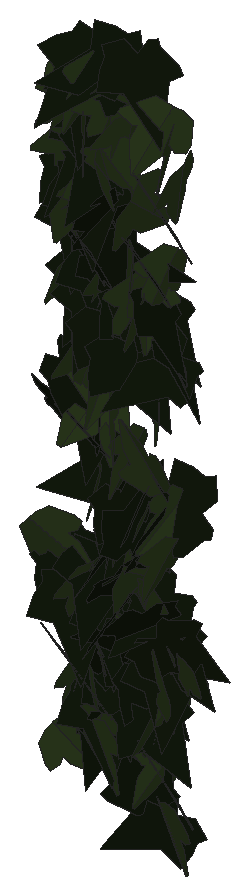
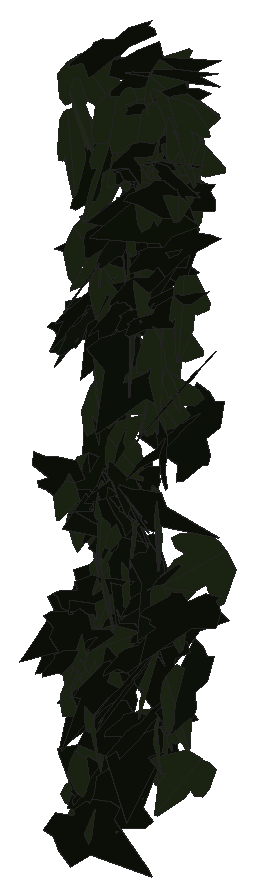
# SketchUp Ruby script. Lengths in inches.
U = 1.inch
M = Sketchup.active_model
def pt(a) = Geom::Point3d.new(a.map { |v| v * U })
def face(e, loops, mat)
  f = e.add_face(loops[0].map { |a| pt(a) })
  loops[1..].each { |l| e.add_face(l.map { |a| pt(a) }).erase! }
  f.material = f.back_material = mat if mat
  f
end
# faces: each face lists its corners as indices into pts; further lists are holes
def faces(e, pts, list, mat = nil) = list.each { |f| face(e, (f[0].is_a?(Array) ? f : [f]).map { |l| l.map { |i| pts[i] } }, mat) }
# xy, xz, yz: faces in a plane at the given z, y or x. An outline is a flat list of corners, or four numbers for a rectangle; further outlines are holes
def ring(l) = l.size == 4 ? [[l[0], l[1]], [l[2], l[1]], [l[2], l[3]], [l[0], l[3]]] : l.each_slice(2).to_a
def flat(e, list, mat, &to3) = list.each { |f| face(e, (f[0].is_a?(Array) ? f : [f]).map { |l| ring(l).map { |u, v| to3.(u, v) } }, mat) }
def xy(e, z, list, mat = nil) = flat(e, list, mat) { |x, y| [x, y, z] }
def xz(e, y, list, mat = nil) = flat(e, list, mat) { |x, z| [x, y, z] }
def yz(e, x, list, mat = nil) = flat(e, list, mat) { |y, z| [x, y, z] }
def lines(e, pts, list) = list.each { |a, b| e.add_line(pt(pts[a]), pt(pts[b])) }
# prism: a flat outline (further loops are holes) pulled along v
def prism(e, loops, v, mat = nil)
  f = face(e, loops, mat); d = Geom::Vector3d.new(v.map { |x| x * U })
  f.pushpull(f.normal.samedirection?(d) ? d.length : -d.length)
end
def box(e, o, s, mat = nil) = prism(e, [[o, [o[0] + s[0], o[1], o[2]], [o[0] + s[0], o[1] + s[1], o[2]], [o[0], o[1] + s[1], o[2]]]], [0, 0, s[2]], mat)
def at(x, y, z, deg = 0) = Geom::Transformation.translation(pt([x, y, z])) * Geom::Transformation.rotation(ORIGIN, Z_AXIS, deg.degrees)
def axes(o, x, y, z) = Geom::Transformation.new([*x, 0, *y, 0, *z, 0, *pt(o).to_a, 1])
def part(name) = M.definitions.add(name)
# library, detail: a bought-in or finely detailed component or shape, given as its bounding box
def library(name, o, s) = part(name).tap { |d| box(d.entities, o, s) }
def detail(e, o, s) = box(e.add_group.entities, o, s)
def put(e, d, t, mat = nil) = e.add_instance(d, t).tap { |i| i.material = mat if mat }
def group(e, t, mat = nil) = e.add_group.tap { |g| g.transformation = t; g.material = mat if mat }.entities
root = M.entities
M.materials.add("efeu1").color = [18, 25, 13]
M.materials.add("efeu2").color = [43, 57, 29]
c1 = part("ivyleaf_10")
p = [[0,0.5,-0.03],[-0.0625,2.02,-0.43],[-0.19,2.01,-0.46],[-0.54,1.05,-0.29],[-0.52,0.625,-0.18],[-0.83,0.76,-0.28],
  [-1.16,0.64,-0.33],[-1.15,0.33,-0.24],[-0.77,-0.39,0.02],[-0.3,-0.51,0.16],[0.04,-0.48,0.23],[-0.02,2.01,-0.4375],
  [-0.06,2.01,-0.43],[0.04,-0.49,0.23],[0.67,-0.49,0.14],[1.38,0.36,-0.2],[1.375,0.51,-0.24],[0.81,0.65,-0.19],
  [0.62,0.59,-0.15],[0.6,1.09,-0.28],[0.5,1.23,-0.31]]
faces(c1.entities,p,[[0,1,2,3,4,5,6,7,8,9,10],[11,12,0,13,14,15,16,17,18,19,20]],"efeu2")
c2 = part("ivyleaf_9")
p = [[1.54,2.16,1.25],[1.36,2.04,1.19],[-0.21,0.99,0.68],[-0.71,1.11,0.82],[-0.85,0.86,0.67],[-0.8,0.17,0.21],
  [-0.9,-0.01,0.1],[-0.67,-0.16,-0.02],[-0.08,-0.08,-0.05],[-0.03,-0.6,-0.4],[0.65,-0.88,-0.66],[0.83,-0.6,-0.49],
  [1.29,-0.42,-0.43],[1.8125,-0.07,-0.26],[1.21,0.44,0.15]]
faces(c2.entities,p,[[0,1,2,3,4,5,6,7,8,9,10,11,12,13,14]],"efeu1")
put(root,c1,axes([527.49,134.28,199.55],[0.10331,-0.77036,-0.31589],[0.02742,0.32128,-0.77456],[0.83216,0.08505,0.06474]))
put(root,c1,axes([527.53,134.26,204.45],[0.00296,-0.85137,0.05429],[0.01786,-0.05421,-0.85119],[0.85291,0.00408,0.01763]))
put(root,c1,axes([527.09,133.73,191.82],[-0.55023,-0.01152,-0.61627],[0.61539,0.03637,-0.55013],[0.0348,-0.82536,-0.01563]))
put(root,c2,axes([527.21,134.57,190.82],[0.02669,-0.53096,-0.58579],[0.07368,0.58524,-0.5271],[0.78717,-0.03678,0.0692]))
put(root,c1,axes([527.72,134.58,204.76],[-0.5819,-0.55056,0.2142],[-0.09039,-0.21415,-0.79598],[0.58381,-0.58192,0.09026]))
put(root,c1,axes([527.43,134.8,205.12],[0.84438,-0.03795,0.0025],[0.00327,0.01701,-0.84506],[0.03789,0.84422,0.01714]))
put(root,c1,axes([527.77,134.18,203.35],[-0.60526,-0.56127,0.00643],[-0.00507,-0.00399,-0.82544],[0.56128,-0.60528,-0.00052]))
put(root,c1,axes([527.49,133.99,185.72],[0.32694,0.47097,0.47558],[0.1738,0.4514,-0.5665],[-0.64636,0.3596,0.08824]))
put(root,c2,axes([527.64,134.87,201.06],[-0.28917,-0.75904,-0.0645],[0.0197,0.06152,-0.81225],[0.76152,-0.28981,-0.00348]))
put(root,c2,axes([527.11,134.03,195.4],[0.59961,-0.41124,0.45427],[0.37216,-0.26053,-0.72708],[0.48681,0.70571,-0.0037]))
put(root,c1,axes([527.89,134.27,187.93],[0.213,-0.80801,0.14369],[0.05539,-0.13396,-0.83539],[0.81881,0.21925,0.01913]))
put(root,c2,axes([527.89,135,199.15],[-0.33172,-0.70773,0.18093],[-0.02622,-0.18705,-0.77973],[0.73002,-0.32831,0.05421]))
put(root,c2,axes([527.34,134.16,188.06],[0.53366,-0.51151,0.41089],[0.28566,-0.29567,-0.73909],[0.59065,0.60515,-0.0138]))
put(root,c2,axes([527.65,133.8,196.87],[0.5477,-0.49041,-0.45193],[-0.19676,0.43995,-0.71585],[0.6372,0.55737,0.16741]))
put(root,c2,axes([527.68,134.5,202.52],[-0.11047,-0.63485,-0.51519],[0.22003,0.47761,-0.63572],[0.78743,-0.22252,0.10536]))
put(root,c1,axes([528.34,134.28,186.85],[-0.07324,0.12878,-0.83192],[-0.32133,0.76756,0.14711],[0.77809,0.32911,-0.01755]))
put(root,c1,axes([528.1875,134.55,193.38],[0.34283,-0.596,-0.44686],[-0.15045,0.42638,-0.6841],[0.72956,0.368,0.06891]))
put(root,c2,axes([527.83,134.27,190],[-0.22233,-0.79633,-0.23959],[0.10442,0.21931,-0.82582],[0.82501,-0.24236,0.03995]))
put(root,c2,axes([528.625,134.9,193.3125],[-0.61958,0.04282,0.46131],[-0.46161,0.00845,-0.62077],[-0.0394,-0.77241,0.01878]))
put(root,c2,axes([528.22,134.72,203.05],[-0.78111,-0.17497,-0.20759],[0.20422,0.03799,-0.80043],[0.1789,-0.80733,0.00732]))
put(root,c2,axes([528.2,134.53,205.75],[-0.69733,-0.48736,0.10601],[0.07458,-0.28207,-0.80617],[0.49315,-0.64649,0.27182]))
put(root,c1,axes([528.1875,134.14,190.65],[0.02802,-0.80758,0.08612],[-0.00555,-0.08636,-0.80803],[0.81214,0.02727,-0.00849]))
put(root,c2,axes([528.42,134.15,194.625],[0.04968,-0.09958,0.80488],[-0.177,0.78562,0.10812],[-0.79146,-0.18194,0.02634]))
put(root,c2,axes([527.92,134.94,203.9375],[-0.17494,-0.77201,-0.2741],[0.06505,0.2663,-0.79157],[0.81664,-0.18659,0.00434]))
put(root,c2,axes([527.87,134.95,195.23],[-0.03168,-0.79066,0.24981],[0.03349,-0.25101,-0.7902],[0.82851,-0.02008,0.0415]))
put(root,c1,axes([528.06,134.42,204.07],[-0.18171,0.64404,-0.48709],[0.08272,-0.4818,-0.6679],[-0.80325,-0.19531,0.04141]))
put(root,c2,axes([528.11,134.74,205],[-0.3204,-0.76889,-0.04698],[0.00681,0.04805,-0.83289],[0.77029,-0.32024,-0.01217]))
put(root,c1,axes([528.39,134.98,204.6],[-0.41538,-0.68563,0.16225],[-0.05821,-0.1543,-0.8011],[0.70216,-0.4184,0.02957]))
put(root,c2,axes([528.38,134.74,203],[-0.66306,-0.47663,0.15068],[-0.00707,-0.24134,-0.7945],[0.49983,-0.6357,0.18866]))
put(root,c1,axes([528.22,134.37,205.36],[0.01143,-0.59414,0.59444],[0.14879,-0.58367,-0.58624],[0.82718,0.1132,0.09724]))
put(root,c1,axes([528.4,134.3,202.2],[-0.13464,-0.76169,0.27538],[-0.05587,-0.26975,-0.77346],[0.80801,-0.14557,-0.0076]))
put(root,c1,axes([527.87,134.5,197.25],[0.49523,-0.3055,0.55505],[0.50745,-0.23056,-0.57966],[0.37935,0.70723,0.05079]))
put(root,c2,axes([527.99,134.82,185.7],[0.07076,-0.61448,0.47429],[0.01943,-0.4747,-0.61791],[0.77599,0.06792,-0.02778]))
put(root,c2,axes([528.48,133.92,190.74],[0.03381,0.58839,0.52367],[0.03509,0.52251,-0.58935],[-0.78689,0.04858,-0.00378]))
put(root,c1,axes([528.24,133.45,202],[-0.16552,-0.50699,-0.67074],[0.34536,0.58229,-0.52536],[0.76659,-0.3718,0.09185]))
put(root,c1,axes([528.49,133.87,197.63],[-0.17434,-0.84804,-0.19718],[0.0386,0.19337,-0.86577],[0.8698,-0.17856,-0.0011]))
put(root,c2,axes([528.08,133.88,201.51],[0.65023,0.20008,0.46236],[0.27221,0.4957,-0.59732],[-0.42392,0.62519,0.32564]))
put(root,c1,axes([528.47,134.39,188.63],[-0.37886,0.63679,0.1376],[-0.08096,0.11192,-0.74087],[-0.64644,-0.38722,0.01215]))
put(root,c2,axes([528.41,133.56,200.72],[0.68456,-0.01253,-0.44843],[-0.44753,0.03763,-0.68423],[0.03109,0.81749,0.02462]))
put(root,c1,axes([528.65,134.04,196.22],[0.80537,0.17384,-0.4092],[-0.3993,-0.08949,-0.82391],[-0.1955,0.89892,-0.00289]))
put(root,c2,axes([528.91,134.82,205.47],[-0.42071,-0.22964,0.69068],[-0.57614,-0.38244,-0.47809],[0.44479,-0.71259,0.03401]))
put(root,c2,axes([528.37,134.46,190.83],[-0.13954,-0.79423,0.16324],[-0.01463,-0.16315,-0.80628],[0.8107,-0.13965,0.01355]))
put(root,c1,axes([528.79,134.01,186.54],[-0.69073,-0.21362,0.19897],[-0.18861,-0.06354,-0.72299],[0.22281,-0.716,0.0048]))
put(root,c2,axes([528.38,134.61,199.79],[-0.15454,-0.77185,-0.17177],[0.01762,0.17161,-0.78701],[0.79054,-0.15472,-0.01604]))
put(root,c2,axes([528.51,134.5,198.875],[-0.34937,-0.72606,0.10089],[-0.01729,-0.10357,-0.80522],[0.73283,-0.34859,0.0291]))
put(root,c1,axes([528.59,134.52,199.6],[0.20606,-0.76636,0.15382],[0.04655,-0.14676,-0.79355],[0.78026,0.21115,0.00672]))
put(root,c2,axes([528.27,135.1,187.23],[0.18199,-0.75284,-0.09867],[-0.01981,0.09673,-0.77452],[0.75902,0.18303,0.00344]))
put(root,c2,axes([528.35,135.03,189.42],[-0.04621,-0.78724,-0.05396],[0.0144,0.05321,-0.78851],[0.78895,-0.04708,0.01123]))
put(root,c2,axes([528.39,134.1,202.41],[-0.48061,-0.4786,-0.46938],[0.40857,0.24874,-0.67197],[0.53145,-0.62404,0.09213]))
put(root,c2,axes([528.95,134.05,189.04],[0.25419,0.56591,-0.44058],[-0.29365,-0.34433,-0.6117],[-0.65432,0.37437,0.10337]))
put(root,c1,axes([528.81,134.52,204.75],[-0.22226,-0.77281,0.28209],[0.01245,-0.29533,-0.79928],[0.8226,-0.20434,0.08831]))
put(root,c2,axes([528.73,134.53,203.16],[-0.32063,-0.74132,0.36975],[-0.11782,-0.35165,-0.80718],[0.82,-0.34039,0.0286]))
put(root,c2,axes([528.57,134.42,187.04],[-0.19649,-0.7341,-0.27689],[0.11081,0.25662,-0.75898],[0.77672,-0.22232,0.03824]))
put(root,c1,axes([528.86,134.22,196.91],[0.12138,0.66374,-0.44421],[-0.15164,-0.42198,-0.67197],[-0.78414,0.18435,0.06119]))
put(root,c1,axes([529.12,134.69,204.49],[-0.52872,-0.61792,0.22347],[-0.14321,-0.17157,-0.81324],[0.64129,-0.54777,0.00264]))
put(root,c1,axes([528.73,133.92,186.18],[-0.60149,0.35762,-0.39824],[0.30581,-0.26203,-0.6972],[-0.43928,-0.6721,0.05992]))
put(root,c1,axes([529.18,133.54,203.23],[-0.39949,0.48953,0.5391],[-0.32499,0.43041,-0.63166],[-0.65166,-0.51475,-0.01547]))
put(root,c2,axes([529.01,134.21,197.0625],[0.32016,0.68552,0.29584],[0.06964,0.29307,-0.75447],[-0.74338,0.3227,0.05673]))
put(root,c2,axes([528.72,135.28,188.22],[0.11446,-0.73491,0.16893],[0.02908,-0.16643,-0.74377],[0.75352,0.11806,0.00305]))
put(root,c2,axes([528.77,133.45,201.3],[0.27252,0.2953,0.71633],[0.47915,0.53251,-0.40181],[-0.60889,0.55121,0.00442]))
put(root,c2,axes([529.21,134.8,194.14],[-0.55414,0.35619,-0.41437],[0.33438,-0.2457,-0.65838],[-0.43216,-0.64684,0.02191]))
put(root,c2,axes([529.15,134.2,186.55],[0.51076,0.5818,-0.35925],[-0.23423,-0.27241,-0.77418],[-0.6424,0.5619,-0.00335]))
put(root,c2,axes([528.72,134.98,188.14],[0.37089,-0.68105,-0.15357],[-0.07487,0.13409,-0.77549],[0.69412,0.37837,-0.00159]))
put(root,c1,axes([529.13,134.32,197.92],[0.38709,-0.6086,-0.35473],[-0.03601,0.38713,-0.70349],[0.70351,0.35468,0.15918]))
put(root,c1,axes([528.71,134.15,195.85],[0.5952,-0.25977,0.46688],[0.45467,-0.12079,-0.64684],[0.2806,0.74676,0.05778]))
put(root,c2,axes([529.51,133.74,190.14],[-0.40073,0.67454,-0.16754],[0.07948,-0.14765,-0.78456],[-0.69047,-0.40848,0.00692]))
put(root,c2,axes([529.59,134.77,184.25],[0.28531,-0.06019,0.74043],[-0.7075,0.21983,0.29049],[-0.22651,-0.76244,0.02531]))
put(root,c1,axes([529.08,133.9,203.47],[-0.6673,-0.33583,-0.36302],[0.32096,0.16974,-0.74701],[0.37623,-0.74045,-0.0066]))
put(root,c1,axes([529.32,133.89,192.75],[0.41712,-0.52482,-0.47962],[-0.07397,0.52102,-0.63445],[0.70711,0.36409,0.21656]))
put(root,c2,axes([529.37,134.68,193.375],[-0.65419,0.00995,-0.3998],[0.39906,-0.03418,-0.65382],[-0.02631,-0.76592,0.02398]))
put(root,c1,axes([529.31,134.71,194.68],[0.10312,-0.60012,0.49082],[0.15043,-0.47025,-0.60657],[0.76054,0.17438,0.05342]))
put(root,c1,axes([529.5,134.29,204.34],[-0.18911,-0.81721,-0.02621],[0.01922,0.02245,-0.8387],[0.81741,-0.18959,0.01365]))
put(root,c2,axes([528.89,133.88,200.47],[0.22479,0.1624,-0.82068],[0.44455,0.69669,0.25963],[0.7087,-0.48853,0.09744]))
put(root,c2,axes([529.2,134.55,198.83],[0.23386,-0.7372,-0.23846],[-0.07249,0.22717,-0.77341],[0.77141,0.24484,-0.00039]))
put(root,c2,axes([529.62,133.57,191.32],[0.17173,0.74034,0.09604],[0.02002,0.09395,-0.75999],[-0.74627,0.17288,0.00171]))
put(root,c2,axes([529.16,133.77,198.74],[-0.00777,-0.50441,-0.69018],[0.28001,0.65063,-0.47866],[0.8077,-0.23041,0.1593]))
put(root,c1,axes([530.19,134.61,188.51],[-0.42399,0.08487,-0.70567],[-0.68211,0.18232,0.43176],[0.19973,0.8028,-0.02346]))
put(root,c1,axes([529.71,134.52,199.37],[-0.08622,-0.75373,0.44267],[0.04952,-0.44831,-0.7537],[0.87271,-0.04903,0.08651]))
put(root,c2,axes([529.4,134.14,193.41],[0.17468,-0.61743,-0.53459],[-0.04776,0.53802,-0.637],[0.81531,0.1638,0.07722]))
put(root,c2,axes([529.85,134.89,192.6875],[-0.5746,-0.53973,0.10431],[-0.07848,-0.06881,-0.78833],[0.54409,-0.57993,-0.00355]))
put(root,c1,axes([529.74,133.92,200.57],[0.56881,-0.53982,-0.22905],[-0.04013,0.28252,-0.7655],[0.58503,0.54423,0.17019]))
put(root,c1,axes([529.79,134.8,191.02],[0.47781,-0.59829,-0.11606],[-0.05907,0.10131,-0.76548],[0.60657,0.48115,0.01688]))
put(root,c1,axes([529.78,134.34,190.6875],[-0.71981,0.23872,-0.05263],[0.05258,-0.00863,-0.75832],[-0.23873,-0.72168,-0.00835]))
put(root,c2,axes([529.59,134.64,188.07],[0.28347,-0.52808,-0.61317],[-0.24676,0.56235,-0.59839],[0.77068,0.37429,0.03394]))
put(root,c2,axes([530.31,135.08,183.79],[0.00662,0.04927,-0.80859],[-0.49783,-0.63767,-0.04293],[-0.63907,0.49724,0.02507]))
put(root,c1,axes([529.82,133.78,191.45],[-0.0032,-0.47373,-0.67238],[0.11953,0.66498,-0.46909],[0.81377,-0.09954,0.06626]))
put(root,c1,axes([529.92,134.45,192.89],[0.14162,-0.62822,-0.41581],[-0.04045,0.41614,-0.6425],[0.75228,0.14064,0.04373]))
put(root,c2,axes([529.6,133.99,192.57],[-0.06921,0.67805,0.50529],[0.05439,-0.50236,0.68157],[0.84386,0.08798,-0.00249]))
put(root,c2,axes([529.57,134.54,206.21],[0.0314,-0.81112,-0.24453],[0.09662,0.24653,-0.80535],[0.84165,0.00196,0.10158]))
put(root,c2,axes([529.36,134.37,200.77],[0.44582,-0.5495,0.46515],[0.30818,-0.3488,-0.70741],[0.65065,0.54172,0.01634]))
put(root,c2,axes([530.23,133.9,190.21],[0.0688,0.67218,-0.35486],[-0.05402,-0.35108,-0.6755],[-0.75817,0.08601,0.01592]))
put(root,c2,axes([530.26,135.01,190.34],[-0.60045,-0.45341,0.18636],[-0.13796,-0.12647,-0.75222],[0.4704,-0.61586,0.01727]))
put(root,c2,axes([529.77,133.82,198.07],[-0.01763,-0.64084,-0.62366],[0.05399,0.62188,-0.64054],[0.89259,-0.05027,0.02642]))
put(root,c1,axes([530.15,133.96,199.29],[0.15823,-0.68342,-0.44499],[-0.00417,0.4526,-0.6966],[0.81551,0.13491,0.08277]))
put(root,c1,axes([530.16,134.93,185.49],[-0.11779,-0.48616,0.52364],[0.01816,-0.53257,-0.49037],[0.71429,-0.06663,0.09882]))
put(root,c2,axes([530.03,133.66,192.34],[-0.24558,-0.30907,0.69732],[0.52049,0.46759,0.39055],[-0.55755,0.57264,0.05746]))
put(root,c1,axes([530.11,133.76,202.42],[-0.09421,-0.63096,-0.69188],[0.12727,0.68029,-0.63772],[0.92769,-0.1574,0.01722]))
put(root,c1,axes([530.38,134.18,196.5],[0.36815,-0.28862,-0.66391],[-0.31718,0.60522,-0.43899],[0.65075,0.45828,0.16163]))
put(root,c1,axes([530.25,134.46,187.02],[0.21491,-0.84956,-0.22005],[-0.06851,0.20962,-0.8762],[0.87492,0.2251,-0.01456]))
put(root,c2,axes([529.66,134.88,194.1],[0.10002,-0.47425,0.62662],[0.34472,-0.54118,-0.46461],[0.70621,0.33134,0.13804]))
put(root,c1,axes([530.63,133.8,194.43],[-0.68112,0.19262,-0.48357],[-0.46509,0.13242,0.70783],[0.23374,0.82476,-0.00071]))
put(root,c1,axes([530.15,134.22,199.67],[0.07549,0.78451,-0.21886],[-0.0079,-0.21909,-0.78803],[-0.81443,0.07484,-0.01264]))
put(root,c2,axes([530.26,133.71,192.2],[0.19228,0.31084,0.71561],[0.19845,0.6933,-0.35447],[-0.75455,0.26155,0.08912]))
put(root,c2,axes([530,134.8,198.85],[0.29941,-0.65219,-0.36735],[-0.05189,0.37661,-0.71093],[0.74673,0.28767,0.09789]))
put(root,c1,axes([530.39,134.77,200.32],[-0.08266,-0.6876,0.47749],[0.1228,-0.48458,-0.67655],[0.82808,0.00323,0.148]))
put(root,c2,axes([530.14,134.26,187.14],[0.01277,-0.53743,-0.54965],[0.0846,0.54737,-0.53324],[0.76407,-0.05162,0.06823]))
put(root,c2,axes([529.96,135.15,198.21],[0.24445,-0.62224,0.46266],[0.2356,-0.40257,-0.6659],[0.73874,0.33429,0.05927]))
put(root,c1,axes([530.68,134.27,204.875],[-0.58237,-0.41135,0.43698],[-0.13019,-0.50781,-0.65153],[0.58584,-0.52176,0.2896]))
put(root,c2,axes([530.81,134.58,197.71],[-0.65572,-0.3778,0.30297],[-0.26059,-0.15458,-0.75676],[0.40819,-0.70559,0.00357]))
put(root,c1,axes([530.4,134.93,204.21],[0.47891,-0.66988,0.24731],[0.1455,-0.19999,-0.82347],[0.6991,0.50052,0.00196]))
put(root,c2,axes([529.95,134.86,185.08],[0.36009,-0.49306,0.55085],[0.31779,-0.44998,-0.61051],[0.66749,0.48022,-0.0065]))
put(root,c1,axes([530.45,134.64,184.06],[-0.67137,0.44723,-0.17969],[0.14977,-0.09927,-0.80669],[-0.45811,-0.68787,-0.0004]))
put(root,c2,axes([530.125,134.8,189.12],[-0.13376,-0.28432,-0.73592],[0.47355,0.56807,-0.30554],[0.63101,-0.48659,0.0733]))
put(root,c2,axes([530.42,134.84,188.44],[-0.22395,-0.75531,-0.10656],[0.03233,0.10156,-0.78781],[0.7621,-0.22626,0.00211]))
put(root,c2,axes([531.26,134.89,193.16],[-0.63865,0.09547,0.5697],[-0.56127,0.09821,-0.64566],[-0.13655,-0.85016,-0.01062]))
put(root,c1,axes([530.67,134.26,187.75],[-0.51561,0.58056,0.05581],[0.03744,-0.0414,0.77647],[0.58203,0.51697,-0.0005]))
put(root,c1,axes([530.69,134.73,193.21],[0.19164,0.41415,-0.66507],[-0.25391,-0.61489,-0.45607],[-0.74119,0.31773,-0.01572]))
put(root,c2,axes([530.29,134.21,199.4],[0.4207,-0.67566,-0.16153],[-0.08779,0.13561,-0.79592],[0.68913,0.42975,-0.00279]))
put(root,c1,axes([530.84,134.7,188.62],[-0.65408,0.26856,0.21992],[-0.22242,0.03592,-0.70537],[-0.26649,-0.68912,0.04894]))
put(root,c1,axes([530.48,135.15,187.46],[-0.15548,-0.04822,0.75409],[0.34052,-0.69175,0.02598],[0.67455,0.33809,0.1607]))
put(root,c1,axes([530.76,134.31,192.16],[0.04952,-0.69104,0.33542],[-0.00303,-0.33629,-0.69239],[0.76814,0.04323,-0.02436]))
put(root,c2,axes([530.27,134.92,197.94],[0.42479,-0.67911,0.09071],[0.03265,-0.08655,-0.80082],[0.68436,0.42565,-0.0181]))
put(root,c2,axes([530.11,134.43,202.2],[0.39682,-0.53999,0.58577],[0.35004,-0.46969,-0.67011],[0.71567,0.52914,0.00297]))
put(root,c2,axes([530.45,134.31,189.37],[-0.01773,-0.07388,-0.76761],[0.17093,0.74834,-0.07597],[0.75197,-0.17184,-0.00083]))
put(root,c1,axes([530.96,134.51,203.22],[0.13227,-0.8257,-0.16833],[0.0008,0.17052,-0.83579],[0.84269,0.12944,0.02721]))
